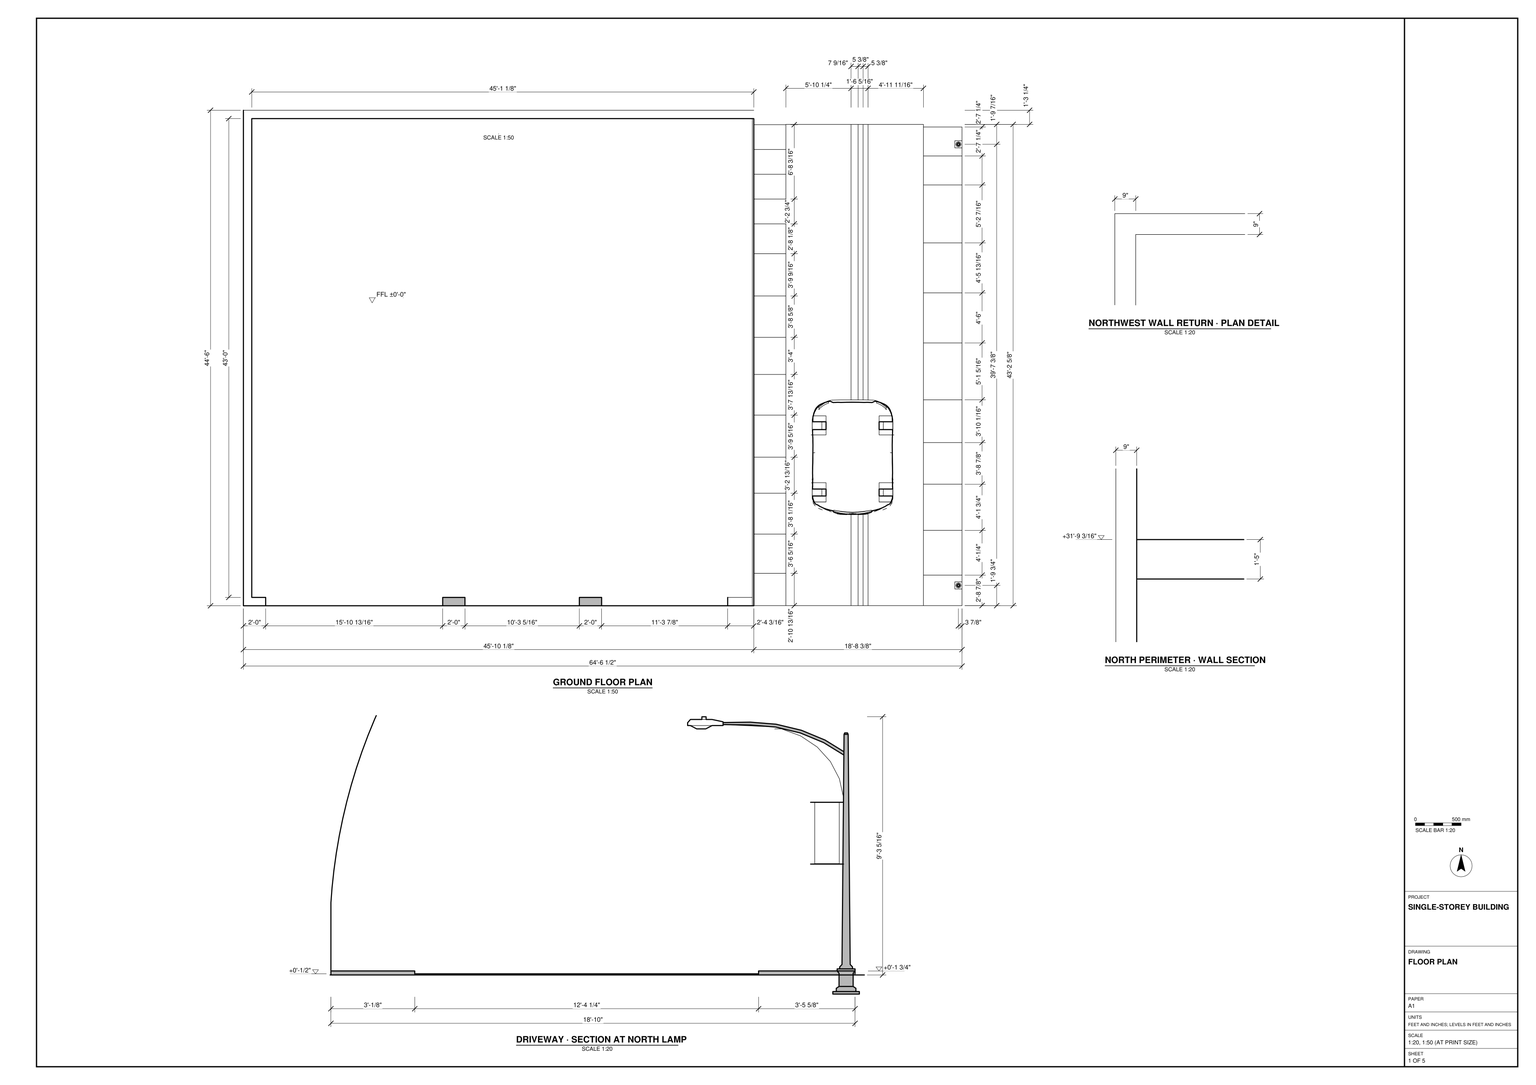
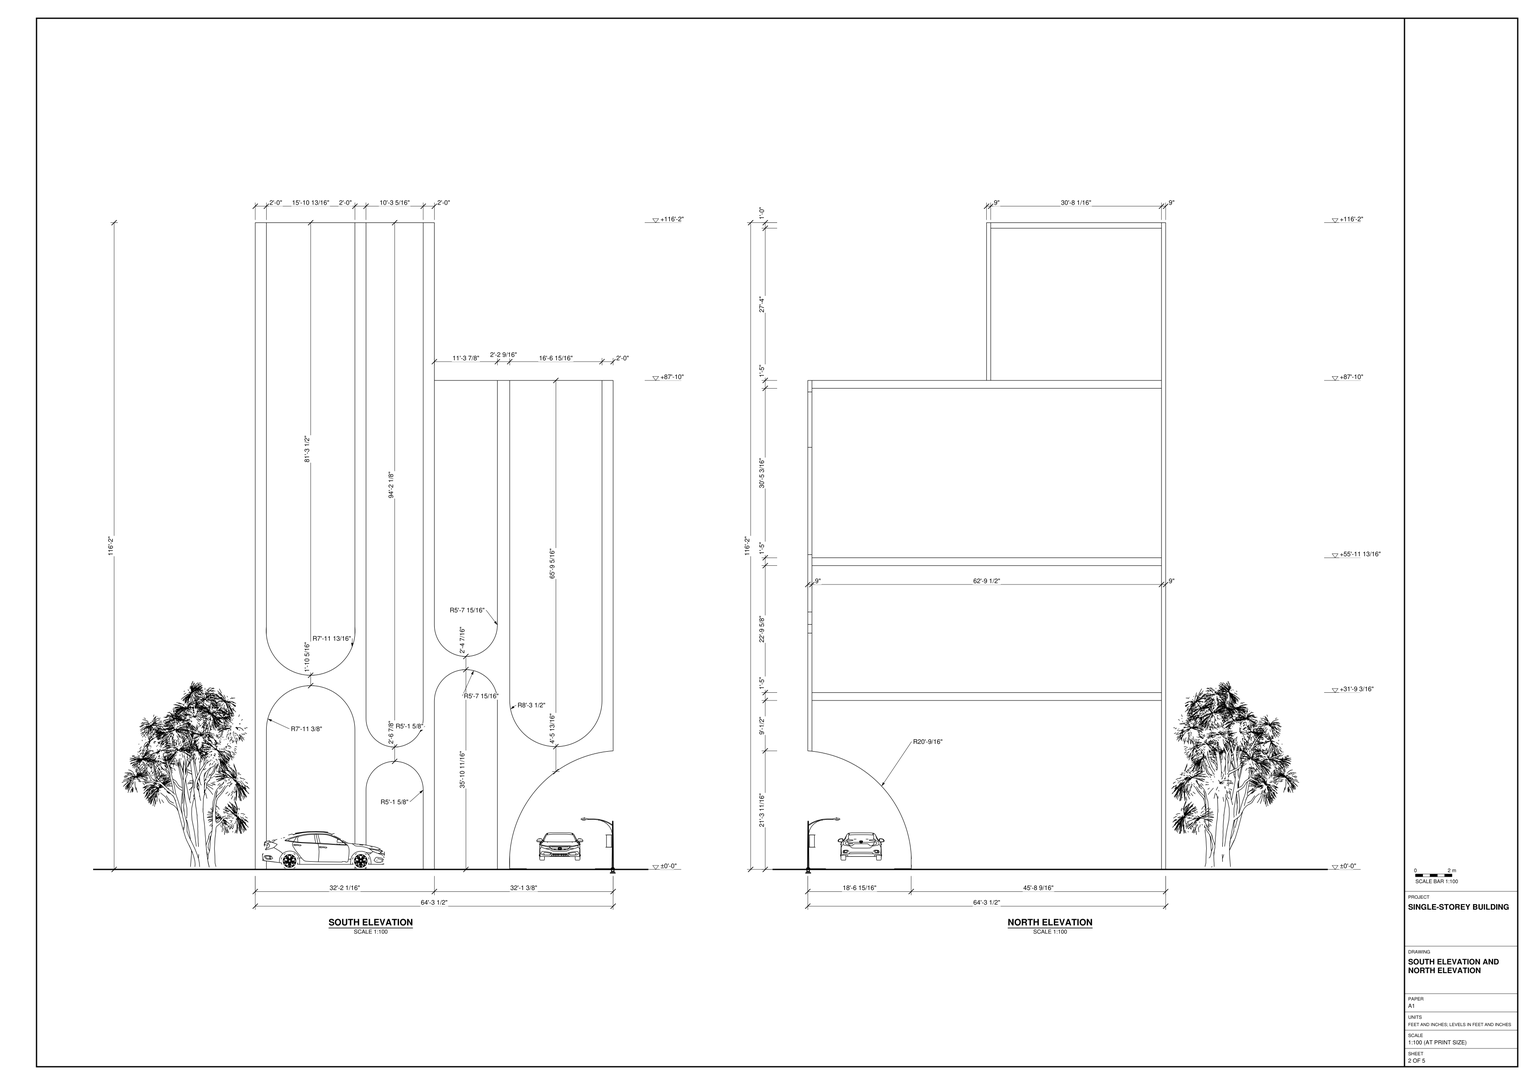
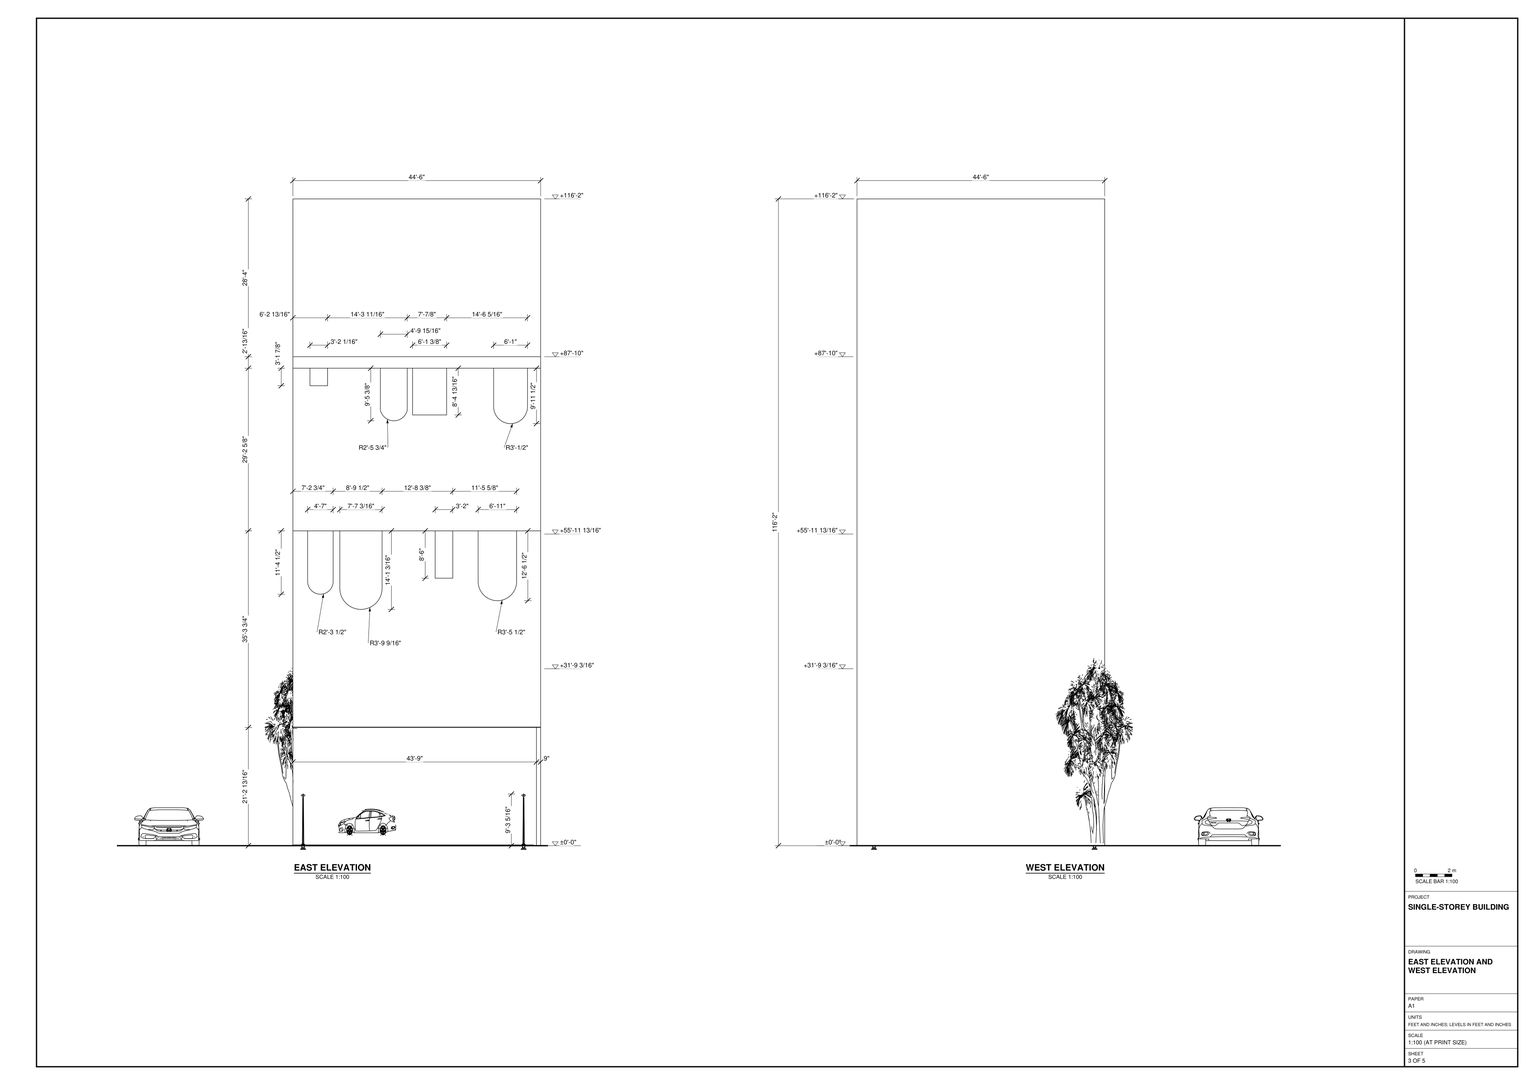
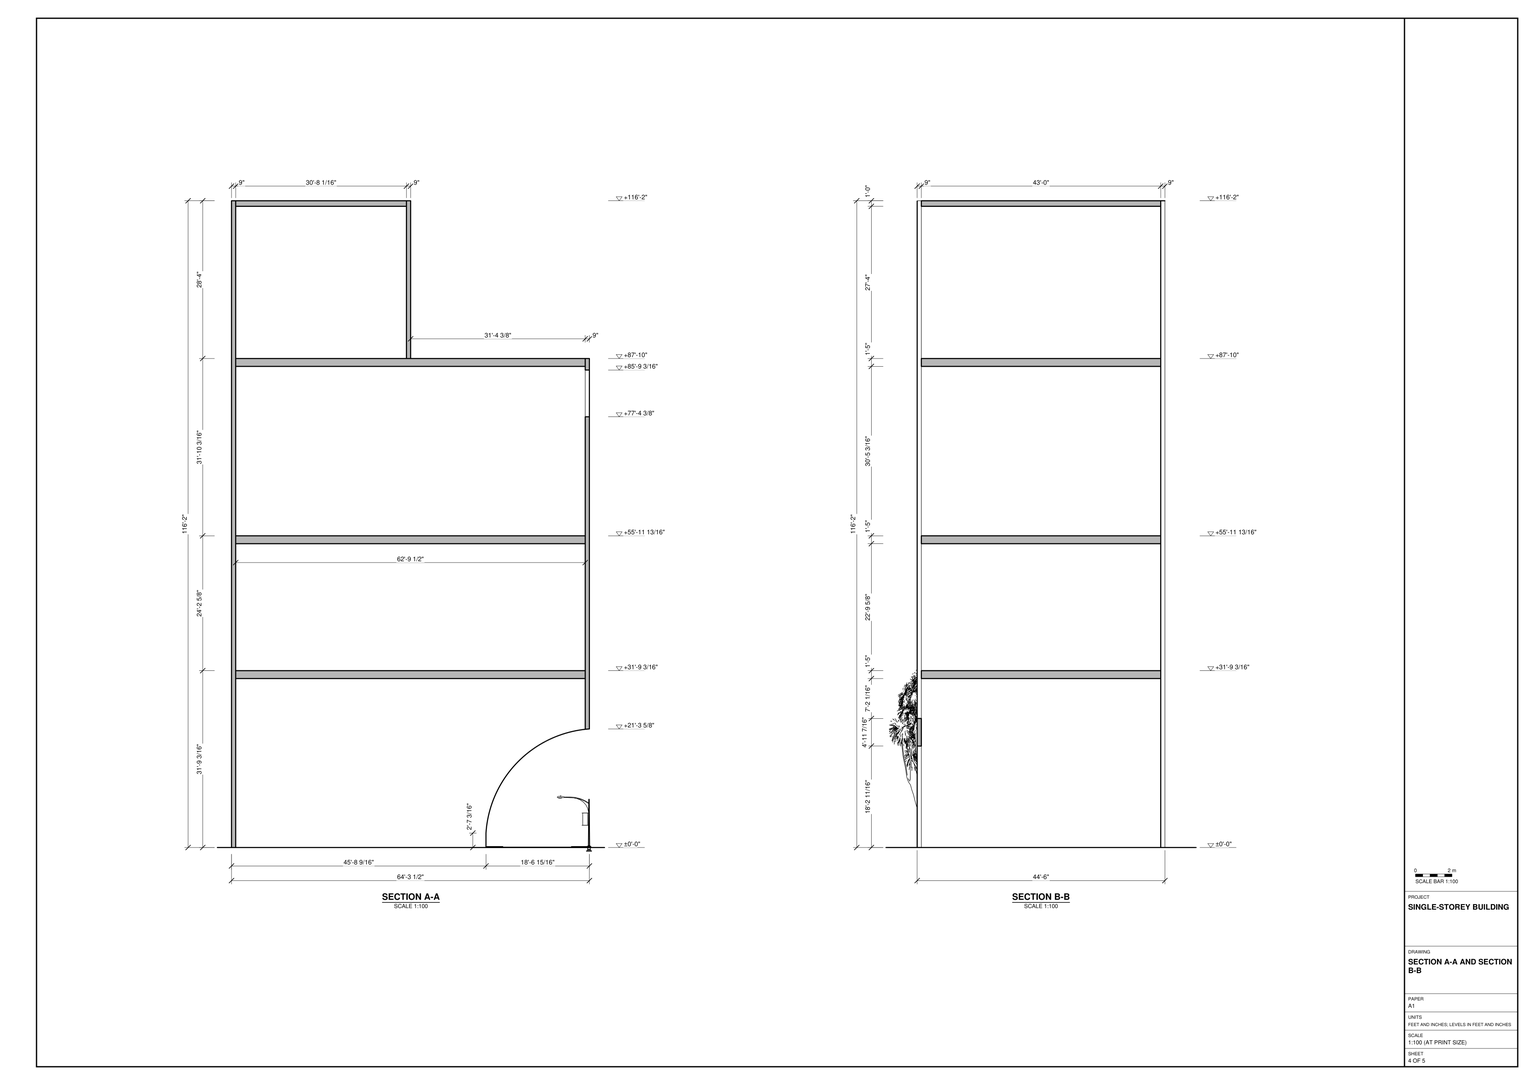
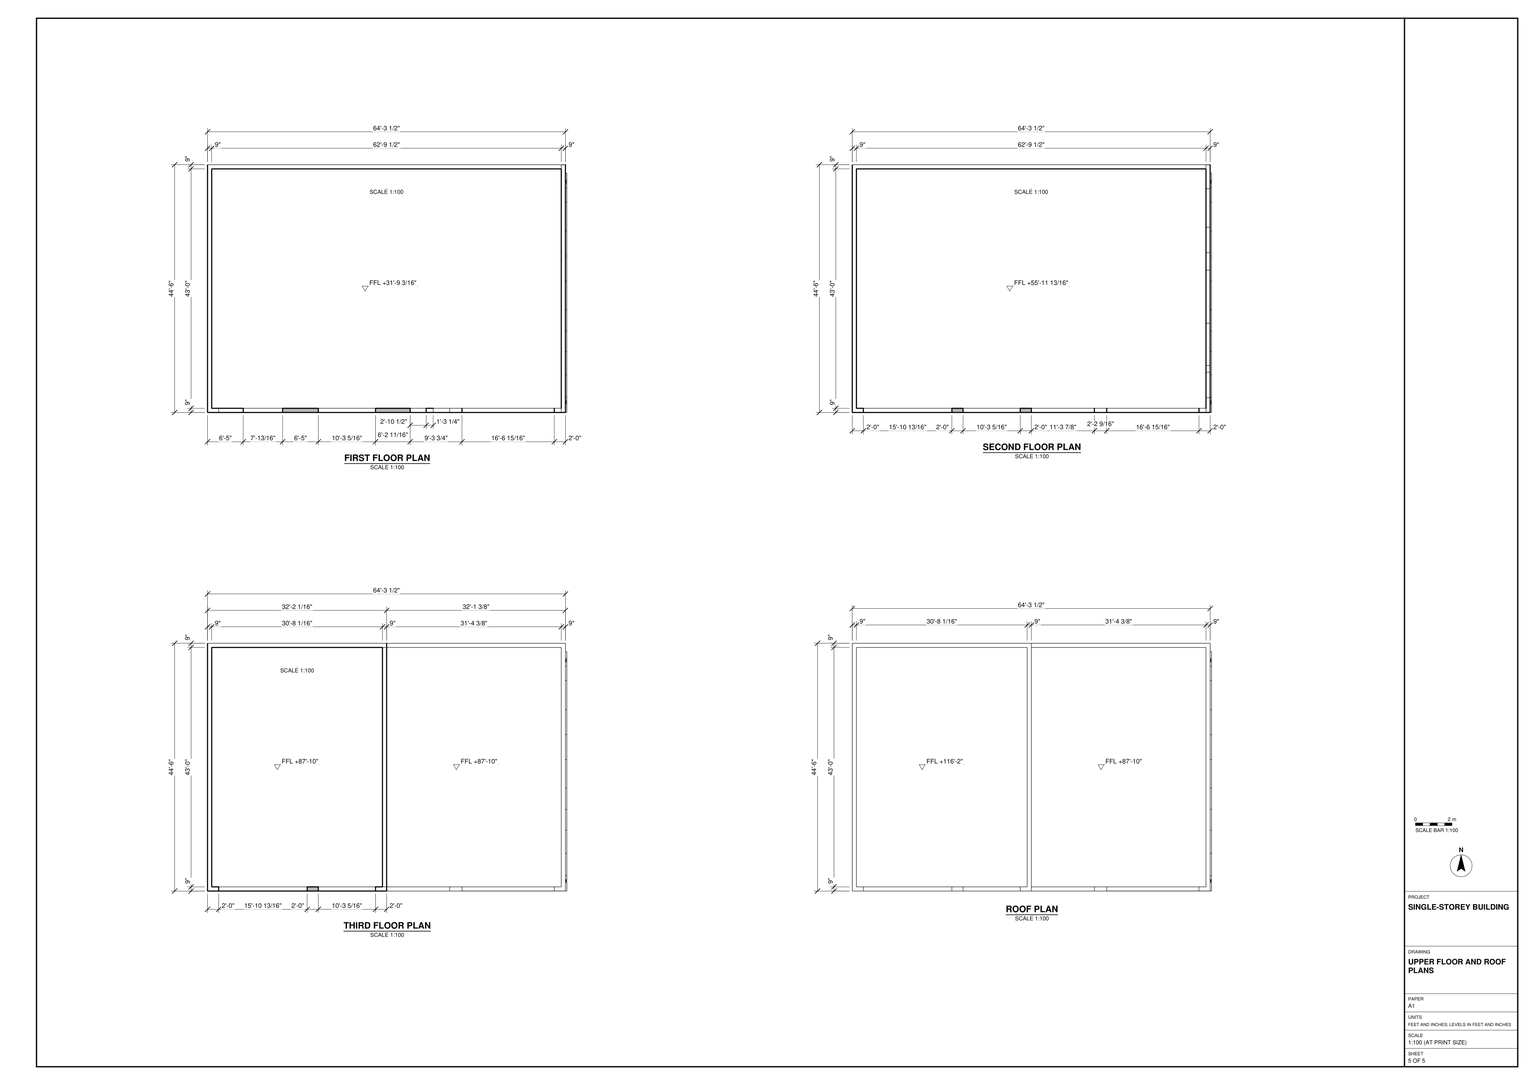
Use task_files/diagram_01.pdf to build the single-storey building and its surrounding site in SketchUp. Work in feet and inches and set the finished ground floor at ±0'-0". The complete model, including the site, must measure 301'-9" along X, 294'-6" along Y and 116'-10 1/4" along Z. Use the ground-floor plan, rather than the overall site extents, to lay out the building footprint.

Model the perimeter walls at their drawn thicknesses, including the northwest wall return. Form the flat roof at two heights, with the taller portion to the west. On the south face, follow the spacing of the long vertical bays, paying particular attention to where their curved ends face one another. Carry the driveway beneath the lower portion of the building and shape the curved clearance profile shown in the north elevation. Include the horizontal slab edges on the north face and the two rows of rounded and square-ended features on the east face. Lay out the driveway edge strips, lamps, cars and planting in the positions shown.

Keep the walls, slabs and roof as separate groups or components, group site elements separately, and use components for repeated parts. Decor and loose site items such as plants, cars and lamps may use any suitable library components. Save one SketchUp model as output_files/stepped_building_and_its_covered_driveway.skp.

# SketchUp Ruby script. Lengths in inches.
U = 1.inch
M = Sketchup.active_model
def pt(a) = Geom::Point3d.new(a.map { |v| v * U })
def face(e, loops, mat)
  f = e.add_face(loops[0].map { |a| pt(a) })
  loops[1..].each { |l| e.add_face(l.map { |a| pt(a) }).erase! }
  f.material = f.back_material = mat if mat
  f
end
# faces: each face lists its corners as indices into pts; further lists are holes
def faces(e, pts, list, mat = nil) = list.each { |f| face(e, (f[0].is_a?(Array) ? f : [f]).map { |l| l.map { |i| pts[i] } }, mat) }
# xy, xz, yz: faces in a plane at the given z, y or x. An outline is a flat list of corners, or four numbers for a rectangle; further outlines are holes
def ring(l) = l.size == 4 ? [[l[0], l[1]], [l[2], l[1]], [l[2], l[3]], [l[0], l[3]]] : l.each_slice(2).to_a
def flat(e, list, mat, &to3) = list.each { |f| face(e, (f[0].is_a?(Array) ? f : [f]).map { |l| ring(l).map { |u, v| to3.(u, v) } }, mat) }
def xy(e, z, list, mat = nil) = flat(e, list, mat) { |x, y| [x, y, z] }
def xz(e, y, list, mat = nil) = flat(e, list, mat) { |x, z| [x, y, z] }
def yz(e, x, list, mat = nil) = flat(e, list, mat) { |y, z| [x, y, z] }
def lines(e, pts, list) = list.each { |a, b| e.add_line(pt(pts[a]), pt(pts[b])) }
# prism: a flat outline (further loops are holes) pulled along v
def prism(e, loops, v, mat = nil)
  f = face(e, loops, mat); d = Geom::Vector3d.new(v.map { |x| x * U })
  f.pushpull(f.normal.samedirection?(d) ? d.length : -d.length)
end
def box(e, o, s, mat = nil) = prism(e, [[o, [o[0] + s[0], o[1], o[2]], [o[0] + s[0], o[1] + s[1], o[2]], [o[0], o[1] + s[1], o[2]]]], [0, 0, s[2]], mat)
def at(x, y, z, deg = 0) = Geom::Transformation.translation(pt([x, y, z])) * Geom::Transformation.rotation(ORIGIN, Z_AXIS, deg.degrees)
def axes(o, x, y, z) = Geom::Transformation.new([*x, 0, *y, 0, *z, 0, *pt(o).to_a, 1])
def part(name) = M.definitions.add(name)
# library, detail: a bought-in or finely detailed component or shape, given as its bounding box
def library(name, o, s) = part(name).tap { |d| box(d.entities, o, s) }
def detail(e, o, s) = box(e.add_group.entities, o, s)
def put(e, d, t, mat = nil) = e.add_instance(d, t).tap { |i| i.material = mat if mat }
def group(e, t, mat = nil) = e.add_group.tap { |g| g.transformation = t; g.material = mat if mat }.entities
root = M.entities
M.materials.add("Asphalt_New").color = [67, 60, 62]
M.materials.add("Color_D01").color = [255, 191, 0]
M.materials.add("Concrete_Aggregate_Smoke").color = [154, 150, 148]
M.materials.add("[Translucent Glass Gray]").color = [128, 128, 128]
c1 = library("006_cordyline_australis",[-46.19,-61.57,-0.26],[141.35,155.27,163.93])
c2 = library("2016+Honda+Civic+LX+Sedan",[0.01,0.03,0.02],[16.17,34.46,10.62])
c3 = part("Lamp01")
xy(c3.entities,28.375,[[9.93,5.75,6.76,6.58,6.65,6.76,6.76,6.93,9.93,7.77,13.1,6.93,13.22,6.76,13.1,6.58]])
xy(c3.entities,31,[[[9.93,0,3.28,1.74,0,6.76,3.28,11.77,9.93,13.52,16.58,11.77,25.88,8.05,25.88,5.46,16.58,1.74],[9.93,1.76,15.52,3.22,17.83,6.76,15.52,10.29,9.93,11.76,4.35,10.29,2.03,6.76,4.35,3.22]]])
xy(c3.entities,35.8,[[[9.93,1.76,15.52,3.22,17.83,6.76,15.52,10.29,9.93,11.76,4.35,10.29,2.03,6.76,4.35,3.22],[10.41,4.875,13.48,8.125]]])
xy(c3.entities,37.92,[[10.41,4.875,13.48,8.125]])
xz(c3.entities,4.875,[[10.41,35.8,13.48,37.92]])
xz(c3.entities,8.125,[[10.41,35.8,13.48,37.92]])
yz(c3.entities,10.41,[[4.875,35.8,8.125,37.92]])
yz(c3.entities,13.48,[[4.875,35.8,8.125,37.92]])
yz(c3.entities,25.88,[[5.46,31,8.05,31,8.05,33.25,7.6,33.86,6.76,33.98,5.92,33.86,5.46,33.25]])
p = [[9.93,1.76,31],[4.35,3.22,31],[6.76,6.58,28.375],[9.93,5.75,28.375],[15.52,3.22,31],[13.1,6.58,28.375],
  [2.03,6.76,31],[6.65,6.76,28.375],[17.83,6.76,31],[13.22,6.76,28.375],[4.35,10.29,31],[6.76,6.93,28.375],
  [15.52,10.29,31],[13.1,6.93,28.375],[9.93,11.76,31],[9.93,7.77,28.375],[3.28,1.74,31],[9.93,0,31],
  [9.93,0,33.25],[3.28,1.74,33.25],[16.58,1.74,31],[16.58,1.74,33.25],[0,6.76,31],[0,6.76,33.25],
  [25.88,5.46,31],[25.88,5.46,33.25],[3.28,11.77,31],[3.28,11.77,33.25],[16.58,11.77,33.25],[25.88,8.05,33.25],
  [25.88,8.05,31],[16.58,11.77,31],[9.93,13.52,31],[9.93,13.52,33.25],[9.93,1.76,35.8],[4.35,3.22,35.8],
  [15.52,3.22,35.8],[2.03,6.76,35.8],[25.88,5.92,33.86],[4.35,10.29,35.8],[15.52,10.29,35.8],[25.88,7.6,33.86],
  [9.93,11.76,35.8],[25.88,6.76,33.98],[17.83,6.76,35.8]]
faces(c3.entities,p,[[0,1,2,3],[4,0,3,5],[1,6,7,2],[8,4,5,9],[6,10,11,7],[12,8,9,13],[10,14,15,11],[14,12,13,15],
  [16,17,18,19],[17,20,21,18],[22,16,19,23],[20,24,25,21],[26,22,23,27],[28,29,30,31],[32,26,27,33],[31,32,33,28],
  [19,18,34,35],[18,21,36,34],[23,19,35,37],[21,25,38,36],[27,23,37,39],[40,41,29,28],[33,27,39,42],[28,33,42,40],
  [36,38,43,44],[44,43,41,40]])
c4 = part("Group\#36")
xy(c4.entities,0,[[0,0,1,24]])
c5 = part("ske72")
xz(c5.entities,-89.9,[[0,212.08,0.94,213.7,-0.94,213.7]])
p = [[-1.3,-15.36,199.9],[-1.3,-0.77,190.22],[-1.14,-1.14,190.14],[0,-1.64,188.09],[0,-16.45,197.92],[1.14,-1.14,190.14],
  [1.3,-0.77,190.22],[1.3,-15.36,199.9],[1.14,-1.14,190.46],[0,-1.61,190.78],[-1.14,-1.14,190.46],[0,-33.46,205.5],
  [-1.3,-32.71,207.63],[1.3,-32.71,207.63],[0,-51.48,210.15],[-1.3,-51.1,212.38],[-1.3,-45.5,210.93],[0,-46.07,208.75],
  [1.3,-51.1,212.38],[1.3,-45.5,210.93],[-0.65,-70.04,212.89],[-1.3,-70,214.01],[0,-70.09,211.76],[0.65,-70.04,212.89],
  [1.3,-70,214.01],[-0.94,-89.9,213.7],[0,-89.9,212.08],[-0.47,-89.9,212.89],[0.94,-89.9,213.7]]
faces(c5.entities,p,[[0,1,2,3,4],[4,3,5,6,7],[7,6,8,9,10,1,0],[11,12,0,4],[13,11,4,7],[12,13,7,0],[14,15,16,12,11,17],[18,14,17,11,13,19],
  [15,18,19,13,12,16],[20,21,15,14,22],[23,22,14,18,24],[25,21,20,22,26,27],[26,22,23,24,28],[21,24,18,15],[25,28,24,21]])
put(c5.entities,c3,at(6.76,-115.78,180.3125,90))
g1 = group(c5.entities,at(-9.6875,-9.6875,0))
box(g1,[0,0,0],[19.37,19.37,2])
xy(g1,6.02,[[4.53,4.53,14.84,14.84]])
xy(g1,19.85,[[3.14,3.14,16.24,16.24]])
xz(g1,2.52,[[2.52,2,16.85,4.57]])
xz(g1,3.14,[[3.14,18.21,16.24,19.85]])
xz(g1,4.53,[[[4.53,6.02,14.84,16.43],[6.19,7.6875,13.18,14.77]],[6.19,7.6875,13.18,14.77]])
xz(g1,14.84,[[[4.53,6.02,14.84,16.43],[6.19,7.6875,13.18,14.77]],[6.19,7.6875,13.18,14.77]])
xz(g1,16.24,[[3.14,18.21,16.24,19.85]])
xz(g1,16.85,[[2.52,2,16.85,4.57]])
yz(g1,2.52,[[2.52,2,16.85,4.57]])
yz(g1,3.14,[[3.14,18.21,16.24,19.85]])
yz(g1,4.53,[[[4.53,6.02,14.84,16.43],[6.19,7.6875,13.18,14.77]],[6.19,7.6875,13.18,14.77]])
yz(g1,14.84,[[[4.53,6.02,14.84,16.43],[6.19,7.6875,13.18,14.77]],[6.19,7.6875,13.18,14.77]])
yz(g1,16.24,[[3.14,18.21,16.24,19.85]])
yz(g1,16.85,[[2.52,2,16.85,4.57]])
p = [[2.52,2.52,4.57],[4.53,4.53,6.02],[4.53,14.84,6.02],[2.52,16.85,4.57],[16.85,2.52,4.57],[14.84,4.53,6.02],
  [16.85,16.85,4.57],[14.84,14.84,6.02],[3.14,3.14,18.21],[3.14,16.24,18.21],[4.53,14.84,16.43],[4.53,4.53,16.43],
  [14.84,4.53,16.43],[16.24,3.14,18.21],[14.84,14.84,16.43],[16.24,16.24,18.21]]
faces(g1,p,[[0,1,2,3],[4,5,1,0],[4,6,7,5],[3,2,7,6],[8,9,10,11],[12,13,8,11],[12,14,15,13],[10,9,15,14]])
g2 = group(c5.entities,at(0,-52.25,154.81))
p = [[0,5.0625,53.9],[0,0,53.9],[0,19,48.39],[0,40.79,28.16],[0,31.15,39.63],[0,47.33,14.67],
  [0,50.35,0]]
lines(g2,p,[[0,1],[2,0],[3,4],[4,2],[5,3],[6,5]])
g3 = group(c5.entities,at(-4.68,-4.68,19.85))
xy(g3,184.57,[[4.68,3.18,5.74,3.62,6.18,4.68,5.74,5.74,4.68,6.18,3.62,5.74,3.18,4.68,3.62,3.62]])
xy(g3,185.69,[[4.68,3.64,5.41,3.95,5.72,4.68,5.41,5.41,4.68,5.72,3.95,5.41,3.64,4.68,3.72,4.5,3.95,3.95]])
p = [[4.68,0,1.5625],[1.37,1.37,1.5625],[1.37,1.37,0],[4.68,0,0],[7.99,1.37,1.5625],[7.99,1.37,0],
  [0,4.68,1.5625],[0,4.68,0],[9.36,4.68,1.5625],[9.36,4.68,0],[1.37,7.99,1.5625],[1.37,7.99,0],
  [7.99,7.99,1.5625],[7.99,7.99,0],[4.68,9.36,1.5625],[4.68,9.36,0],[4.68,1.68,3.4375],[2.56,2.56,3.4375],
  [6.8,2.56,3.4375],[1.68,4.68,3.4375],[7.68,4.68,3.4375],[2.56,6.8,3.4375],[6.8,6.8,3.4375],[4.68,7.68,3.4375],
  [4.68,3.18,184.57],[3.62,3.62,184.57],[5.74,3.62,184.57],[3.18,4.68,184.57],[6.18,4.68,184.57],[3.62,5.74,184.57],
  [5.74,5.74,184.57],[4.68,6.18,184.57],[4.68,3.64,185.69],[3.95,3.95,185.69],[5.41,3.95,185.69],[3.72,4.5,185.69],
  [3.64,4.68,185.69],[5.72,4.68,185.69],[3.95,5.41,185.69],[5.41,5.41,185.69],[4.68,5.72,185.69]]
faces(g3,p,[[0,1,2,3],[4,0,3,5],[1,6,7,2],[8,4,5,9],[6,10,11,7],[12,8,9,13],[10,14,15,11],[14,12,13,15],
  [0,16,17,1],[4,18,16,0],[1,17,19,6],[18,4,8,20],[21,10,6,19],[20,8,12,22],[23,14,10,21],[22,12,14,23],
  [16,24,25,17],[18,26,24,16],[17,25,27,19],[18,20,28,26],[27,29,21,19],[20,22,30,28],[21,29,31,23],[23,31,30,22],
  [24,32,33,25],[26,34,32,24],[33,35,36,27,25],[34,26,28,37],[27,36,38,29],[37,28,30,39],[29,38,40,31],[39,30,31,40]])
g4 = group(c5.entities,at(0,-25.94,102.6875))
yz(g4,0,[[3.04,0,20.96,48]])
put(g4,c4,at(-0.5,0,48.25))
put(g4,c4,at(-0.5,0,-0.375))
c6 = part("road")
xy(c6.entities,0,[[0,61.25,879,180.3125],[0,193.18,879,202.26],[0,211.38,879,312.5]],"Asphalt_New")
xy(c6.entities,0,[[0,180.3125,879,193.18],[0,202.26,879,211.38]],"Color_D01")
xy(c6.entities,2.25,[[0,0,58.96,61.25],[58.96,0,130.63,61.25],[130.63,0,205.31,61.25],[205.31,0,271.13,61.25],[271.13,0,347.96,61.25],
  [347.96,0,422.25,61.25],[422.25,0,490,61.25],[490,0,565.64,61.25],[565.64,0,642.8125,61.25],[642.8125,0,697.3125,61.25],
  [697.3125,0,742.61,61.25],[742.61,0,787.91,61.25],[787.91,0,833.2,61.25],[833.2,0,878.5,61.25],[0,312.5,55.73,383],
  [55.73,312.5,137.52,383],[137.52,312.5,221.8,383],[221.8,312.5,297.83,383],[297.83,312.5,375.9,383],[375.9,312.5,479.79,383],
  [479.79,312.5,571.31,383],[571.31,312.5,662.56,383],[662.56,312.5,768.4,383],[768.4,312.5,821.33,383],[821.33,312.5,874.25,383]],"Concrete_Aggregate_Smoke")
xz(c6.entities,0,[[0,0,58.96,2.25],[58.96,0,130.63,2.25],[130.63,0,205.31,2.25],[205.31,0,271.13,2.25],[271.13,0,347.96,2.25],
  [347.96,0,422.25,2.25],[422.25,0,490,2.25],[490,0,565.64,2.25],[565.64,0,604.23,2.25],[604.23,0,642.8125,2.25],
  [642.8125,0,697.3125,2.25],[697.3125,0,742.61,2.25],[742.61,0,787.91,2.25],[787.91,0,833.2,2.25],[833.2,0,878.5,2.25]],"Concrete_Aggregate_Smoke")
xz(c6.entities,61.25,[[0,0,58.96,2.25],[58.96,0,130.63,2.25],[130.63,0,205.31,2.25],[205.31,0,271.13,2.25],[271.13,0,347.96,2.25],
  [347.96,0,422.25,2.25],[422.25,0,490,2.25],[490,0,565.64,2.25],[565.64,0,642.8125,2.25],[642.8125,0,697.3125,2.25],
  [697.3125,0,742.61,2.25],[742.61,0,787.91,2.25],[787.91,0,833.2,2.25],[833.2,0,878.5,2.25]],"Concrete_Aggregate_Smoke")
xz(c6.entities,312.5,[[0,0,55.73,2.25],[55.73,0,137.52,2.25],[137.52,0,221.8,2.25],[221.8,0,297.83,2.25],[297.83,0,373.56,2.25],
  [373.56,0,375.9,2.25],[375.9,0,479.79,2.25],[479.79,0,571.31,2.25],[571.31,0,662.56,2.25],[662.56,0,768.4,2.25],
  [768.4,0,821.33,2.25],[821.33,0,874.25,2.25]],"Concrete_Aggregate_Smoke")
xz(c6.entities,383,[[0,0,55.73,2.25],[55.73,0,137.52,2.25],[137.52,0,221.8,2.25],[221.8,0,297.83,2.25],[297.83,0,375.9,2.25],
  [375.9,0,479.79,2.25],[479.79,0,571.31,2.25],[571.31,0,662.56,2.25],[662.56,0,768.4,2.25],[768.4,0,821.33,2.25],
  [821.33,0,874.25,2.25]],"Concrete_Aggregate_Smoke")
yz(c6.entities,0,[[0,0,61.25,2.25],[312.5,0,383,2.25]],"Concrete_Aggregate_Smoke")
yz(c6.entities,874.25,[[312.5,0,383,2.25]],"Concrete_Aggregate_Smoke")
yz(c6.entities,878.5,[[0,0,61.25,2.25]],"Concrete_Aggregate_Smoke")
# 1 loose lines left out
put(c6.entities,c5,at(36.91,376.45,-15.96))
put(c6.entities,c5,at(842.66,376.45,-15.96))
c7 = library("car",[-0.875,0,0],[16.18,34.45,10.62])
c8 = library("Group\#1",[0,0,0],[771.47,534,1394])
c9 = part("Group\#2")
box(c9.entities,[0,0,0],[753.47,516,17])
box(root,[1479.625,496.08,1382],[368.1,516,12])
xy(root,0,[[0,0,3621,3534]])
xz(root,487.08,[[1494.625,0,1685.42,0,1685.42,300.79,1685.23,306.78,1684.66,312.74,1683.73,318.66,1682.42,324.51,1680.75,330.27,1678.72,335.9,1676.34,341.4,1673.62,346.74,1670.57,351.9,1667.2,356.86,1663.52,361.59,1659.5625,366.09,1655.32,370.33,1650.83,374.29,1646.09,377.96,1641.14,381.33,1635.98,384.38,1630.64,387.1,1625.14,389.48,1619.5,391.51,1613.74,393.1875,1607.9,394.49,1601.98,395.43,1596.01,395.99,1590.02,396.18,1584.03,395.99,1578.0625,395.43,1572.14,394.49,1566.3,393.1875,1560.54,391.51,1554.9,389.48,1549.4,387.1,1544.0625,384.38,1538.9,381.33,1533.95,377.96,1529.21,374.29,1524.72,370.33,1520.48,366.09,1516.52,361.59,1512.84,356.86,1509.47,351.9,1506.42,346.74,1503.7,341.4,1501.32,335.9,1499.29,330.27,1497.62,324.51,1496.3125,318.66,1495.375,312.74,1494.8125,306.78,1494.625,300.79],[1709.42,0,1832.72,0,1832.72,171.3125,1832.59,175.19,1832.23,179.04,1831.625,182.87,1830.78,186.65,1829.7,190.37,1828.39,194.01,1826.85,197.5625,1825.09,201.01,1823.12,204.35,1820.94,207.55,1818.57,210.61,1816.01,213.52,1813.27,216.26,1810.36,218.82,1807.3,221.19,1804.1,223.37,1800.77,225.34,1797.32,227.1,1793.76,228.63,1790.12,229.95,1786.4,231.03,1782.62,231.87,1778.79,232.48,1774.9375,232.84,1771.07,232.96,1767.2,232.84,1763.34,232.48,1759.51,231.87,1755.73,231.03,1752.02,229.95,1748.37,228.63,1744.82,227.1,1741.37,225.34,1738.03,223.37,1734.83,221.19,1731.77,218.82,1728.86,216.26,1726.125,213.52,1723.5625,210.61,1721.19,207.55,1719.01,204.35,1717.04,201.01,1715.28,197.5625,1713.75,194.01,1712.43,190.37,1711.35,186.65,1710.51,182.87,1709.9,179.04,1709.54,175.19,1709.42,171.3125],[1856.72,0,1992.57,0,1992.57,362.73,1992.4375,366.99,1992.04,371.24,1991.37,375.46,1990.4375,379.62,1989.25,383.72,1987.8,387.74,1986.11,391.65,1984.17,395.45,1982,399.13,1979.6,402.66,1976.98,406.03,1974.16,409.23,1971.14,412.25,1967.94,415.07,1964.57,417.68,1961.04,420.08,1957.37,422.26,1953.57,424.19,1949.65,425.89,1945.64,427.33,1941.54,428.52,1937.37,429.45,1933.16,430.12,1928.91,430.52,1924.64,430.66,1920.38,430.52,1916.13,430.12,1911.92,429.45,1907.75,428.52,1903.65,427.33,1899.64,425.89,1895.72,424.19,1891.92,422.26,1888.25,420.08,1884.72,417.68,1881.35,415.07,1878.14,412.25,1875.125,409.23,1872.3,406.03,1869.6875,402.66,1867.29,399.13,1865.12,395.45,1863.18,391.65,1861.49,387.74,1860.04,383.72,1858.85,379.62,1857.92,375.46,1857.25,371.24,1856.85,366.99,1856.72,362.73],[1771.07,263.85,1774.9375,263.97,1778.79,264.34,1782.62,264.94,1786.4,265.79,1790.12,266.87,1793.76,268.18,1797.32,269.72,1800.77,271.48,1804.1,273.45,1807.3,275.625,1810.36,278,1813.27,280.56,1816.01,283.3,1818.57,286.2,1820.94,289.26,1823.12,292.47,1825.09,295.8,1826.85,299.25,1828.39,302.8,1829.7,306.45,1830.78,310.17,1831.625,313.95,1832.23,317.77,1832.59,321.63,1832.72,325.5,1832.72,1394,1709.42,1394,1709.42,325.5,1709.54,321.63,1709.9,317.77,1710.51,313.95,1711.35,310.17,1712.43,306.45,1713.75,302.8,1715.28,299.25,1717.04,295.8,1719.01,292.47,1721.19,289.26,1723.5625,286.2,1726.125,283.3,1728.86,280.56,1731.77,278,1734.83,275.625,1738.03,273.45,1741.37,271.48,1744.82,269.72,1748.37,268.18,1752.02,266.87,1755.73,265.79,1759.51,264.94,1763.34,264.34,1767.2,263.97],[2118.63,264.71,2124.87,264.9,2131.09,265.49,2137.27,266.47,2143.36,267.83,2149.37,269.57,2155.24,271.69,2160.98,274.17,2166.55,277.01,2171.93,280.19,2177.09,283.7,2182.03,287.53,2186.72,291.67,2191.14,296.08,2195.27,300.77,2199.1,305.71,2202.61,310.88,2205.79,316.26,2208.63,321.82,2211.11,327.56,2213.23,333.4375,2214.97,339.4375,2216.34,345.54,2217.3125,351.71,2217.9,357.93,2218.1,364.18,2218.1,1054,2019.16,1054,2019.16,364.18,2019.35,357.93,2019.94,351.71,2020.92,345.54,2022.28,339.4375,2024.02,333.4375,2026.14,327.56,2028.62,321.82,2031.46,316.26,2034.64,310.88,2038.15,305.71,2041.98,300.77,2046.12,296.08,2050.53,291.67,2055.22,287.53,2060.16,283.7,2065.33,280.19,2070.71,277.01,2076.27,274.17,2082.01,271.69,2087.89,269.57,2093.89,267.83,2099.99,266.47,2106.16,265.49,2112.38,264.9],
  [1590.02,418.51,1596.4,418.72,1602.76,419.36,1609.06,420.42,1615.27,421.9,1621.375,423.78,1627.34,426.07,1633.14,428.76,1638.74,431.82,1644.13,435.25,1649.28,439.03,1654.17,443.14,1658.77,447.57,1663.0625,452.3,1667.03,457.31,1670.66,462.5625,1673.93,468.05,1676.83,473.74,1679.34,479.62,1681.46,485.64,1683.17,491.8,1684.46,498.05,1685.34,504.38,1685.42,505.5,1685.42,1394,1494.625,1394,1494.625,505.5,1494.7,504.38,1495.58,498.05,1496.875,491.8,1498.58,485.64,1500.7,479.62,1503.21,473.74,1506.11,468.05,1509.38,462.5625,1513.01,457.31,1516.98,452.3,1521.27,447.57,1525.875,443.14,1530.76,439.03,1535.91,435.25,1541.3,431.82,1546.9,428.76,1552.7,426.07,1558.66,423.78,1564.77,421.9,1570.98,420.42,1577.28,419.36,1583.64,418.72],[1924.64,459.07,1928.91,459.21,1933.16,459.61,1937.37,460.27,1941.54,461.21,1945.64,462.4,1949.65,463.84,1953.57,465.54,1957.37,467.47,1961.04,469.65,1964.57,472.04,1967.94,474.66,1971.14,477.48,1974.16,480.5,1976.98,483.7,1979.6,487.07,1982,490.6,1984.17,494.28,1986.11,498.08,1987.8,501.99,1989.25,506.01,1990.4375,510.11,1991.37,514.27,1992.04,518.49,1992.4375,522.73,1992.57,527,1992.57,1054,1856.72,1054,1856.72,527,1856.85,522.73,1857.25,518.49,1857.92,514.27,1858.85,510.11,1860.04,506.01,1861.49,501.99,1863.18,498.08,1865.12,494.28,1867.29,490.6,1869.6875,487.07,1872.3,483.7,1875.125,480.5,1878.14,477.48,1881.35,474.66,1884.72,472.04,1888.25,469.65,1891.92,467.47,1895.72,465.54,1899.64,463.84,1903.65,462.4,1907.75,461.21,1911.92,460.27,1916.13,459.61,1920.38,459.21]],"[Translucent Glass Gray]")
put(root,c1,axes([1368.03,492.48,5.26],[-1.93979,0,0],[0,1.06864,0],[0,0,2.45283]))
put(root,c2,axes([1750.05,145.2,-0.17],[0,9.24,0],[-7.6551,0,0],[0,0,7.7153]))
put(root,c6,axes([2019.16,487.23,0.5],[0,0.59,0],[0.59,0,0],[0,0,0.5478]))
put(root,c7,axes([2082.54,584.99,20],[6.1908,0,0],[0,3.5979,0],[0,0,5.55502]))
put(root,c8,at(1470.625,487.08,0))
put(root,c9,at(1479.625,496.08,1037))
put(root,c9,at(1479.625,496.08,364.18))
put(root,c9,at(1479.625,496.08,654.82))
